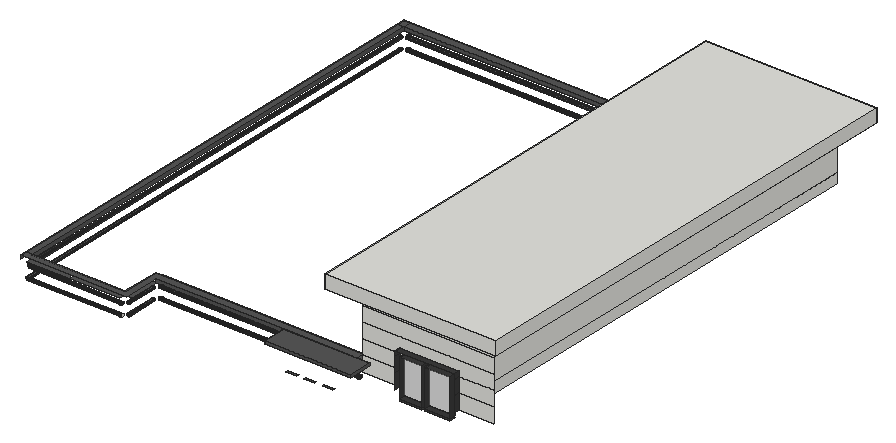
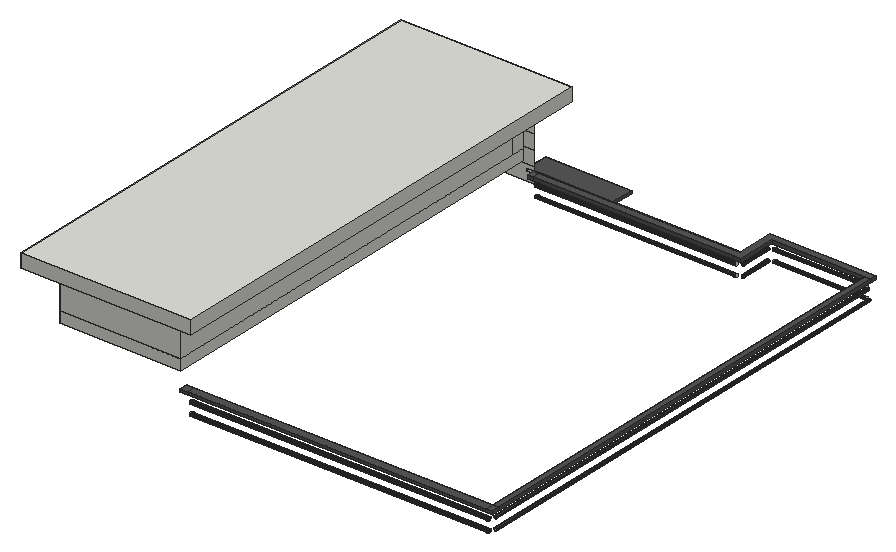
# SketchUp Ruby script. Lengths in inches.
U = 1.inch
M = Sketchup.active_model
def pt(a) = Geom::Point3d.new(a.map { |v| v * U })
def face(e, loops, mat)
  f = e.add_face(loops[0].map { |a| pt(a) })
  loops[1..].each { |l| e.add_face(l.map { |a| pt(a) }).erase! }
  f.material = f.back_material = mat if mat
  f
end
# faces: each face lists its corners as indices into pts; further lists are holes
def faces(e, pts, list, mat = nil) = list.each { |f| face(e, (f[0].is_a?(Array) ? f : [f]).map { |l| l.map { |i| pts[i] } }, mat) }
# xy, xz, yz: faces in a plane at the given z, y or x. An outline is a flat list of corners, or four numbers for a rectangle; further outlines are holes
def ring(l) = l.size == 4 ? [[l[0], l[1]], [l[2], l[1]], [l[2], l[3]], [l[0], l[3]]] : l.each_slice(2).to_a
def flat(e, list, mat, &to3) = list.each { |f| face(e, (f[0].is_a?(Array) ? f : [f]).map { |l| ring(l).map { |u, v| to3.(u, v) } }, mat) }
def xy(e, z, list, mat = nil) = flat(e, list, mat) { |x, y| [x, y, z] }
def xz(e, y, list, mat = nil) = flat(e, list, mat) { |x, z| [x, y, z] }
def yz(e, x, list, mat = nil) = flat(e, list, mat) { |y, z| [x, y, z] }
def lines(e, pts, list) = list.each { |a, b| e.add_line(pt(pts[a]), pt(pts[b])) }
# prism: a flat outline (further loops are holes) pulled along v
def prism(e, loops, v, mat = nil)
  f = face(e, loops, mat); d = Geom::Vector3d.new(v.map { |x| x * U })
  f.pushpull(f.normal.samedirection?(d) ? d.length : -d.length)
end
def box(e, o, s, mat = nil) = prism(e, [[o, [o[0] + s[0], o[1], o[2]], [o[0] + s[0], o[1] + s[1], o[2]], [o[0], o[1] + s[1], o[2]]]], [0, 0, s[2]], mat)
def at(x, y, z, deg = 0) = Geom::Transformation.translation(pt([x, y, z])) * Geom::Transformation.rotation(ORIGIN, Z_AXIS, deg.degrees)
def axes(o, x, y, z) = Geom::Transformation.new([*x, 0, *y, 0, *z, 0, *pt(o).to_a, 1])
def part(name) = M.definitions.add(name)
# library, detail: a bought-in or finely detailed component or shape, given as its bounding box
def library(name, o, s) = part(name).tap { |d| box(d.entities, o, s) }
def detail(e, o, s) = box(e.add_group.entities, o, s)
def put(e, d, t, mat = nil) = e.add_instance(d, t).tap { |i| i.material = mat if mat }
def group(e, t, mat = nil) = e.add_group.tap { |g| g.transformation = t; g.material = mat if mat }.entities
root = M.entities
M.materials.add("[Color M06]").color = [86, 86, 86]
M.materials.add("[Color M07]").color = [58, 58, 58]
M.materials.add("[Translucent Glass Gray]").color = [128, 128, 128]
M.materials["[Translucent Glass Gray]"].alpha = 0.5
M.materials.add("[Wood Fence]").color = [142, 67, 30]
xy(root,343.87,[[283.87,125.84,295.81,128.03],[304,125.84,315.93,128.03],[324.62,125.84,336.56,128.03]],"[Color M06]")
xy(root,347.76,[[3.85,111.5,4.24,637.4375]],"[Color M06]")
xy(root,348.22,[[399.25,141.23,424.3125,147.79],[427.08,141.23,456,147.79]],"[Color M07]")
xy(root,350.29,[[399.25,141.23,424.3125,147.79],[427.08,141.23,456,147.79]],"[Color M07]")
xy(root,366,[[206.23,639.05,209.79,643.61]])
xy(root,366.125,[[[0,113.71,7.24,637.4375],[1.32,218.77,6.25,221.71],[1.32,568.77,6.25,571.71],[1.32,483.08,6.25,486.02],[1.32,393.08,6.25,396.02],[1.32,307.08,6.25,310.02]],[346.24,147.79,352,156.79],[112.36,149.1,120,156.79],[0,637.4375,7.24,646.4375],[[7.24,637.4375,343.33,646.4375],[285.6,637.86,289.17,643.61],[92.17,637.86,95.73,643.55]],
  [343.33,637.4375,352,646.4375]])
xy(root,366.125,[[[7.24,106.4375,112.36,113.71],[52.52,108.5,56.02,112.75]],[112.36,113.71,120,149.1],[120,147.79,346.24,156.79]],"[Color M06]")
xy(root,367.0625,[[266.86,121.03,269.98,140.23],[269.98,128.03,352,140.23]])
xy(root,367.0625,[[263.17,121.03,263.17,147.79,360.875,147.79,360.875,128.03,352,128.03,352,140.23,266.86,140.23,266.86,121.03],[269.98,121.03,360.875,128.03]],"[Color M06]")
xy(root,370,[[0,106.4375,120,106.4375,120,147.79,346.24,147.79,346.24,156.79,112.36,156.79,112.36,113.71,0,113.71],[0,113.71,7.24,637.4375],[263.17,121.03,360.875,147.79],[346.24,147.79,352,156.79],[0,637.4375,7.24,646.4375],
  [7.24,637.4375,343.33,646.4375],[343.33,637.4375,352,646.4375]],"[Color M06]")
xy(root,392.08,[[399.25,141.23,424.3125,147.79],[427.08,141.23,428.9,147.79],[428.9,141.23,456,147.79]],"[Color M07]")
xy(root,394,[[358,155.92,494,637.4375]])
xy(root,397.01,[[394.33,141.23,460.92,147.79]],"[Color M07]")
xy(root,435.0625,[[358,155.92,494,637.4375]])
xy(root,441.0625,[[352,147.79,500,646.4375]])
xy(root,441.0625,[[[325.625,127.92,517.6875,664.0625],[352,147.79,500,646.4375]]],"[Wood Fence]")
xy(root,455.875,[[325.625,127.92,517.6875,664.0625]])
xz(root,111.5,[[4.17,344.78,4.55,344.875,4.9,345.0625,5.18,345.33,5.38,345.67,5.49,346.04,5.5,346.44,5.41,346.82,5.22,347.16,4.95,347.44,4.61,347.65,4.24,347.76,3.85,347.76,3.47,347.67,3.125,347.48,2.84,347.21,2.64,346.88,2.53,346.5,2.52,346.11,2.61,345.73,2.8,345.39,3.07,345.1,3.4,344.9,3.78,344.79]])
xz(root,113.71,[[116.05,345.98,116.46,346,116.84,346.125,117.1875,346.35,117.46,346.65,117.65,347.01,117.73,347.41,117.71,347.82,117.58,348.21,117.36,348.55,117.06,348.82,116.69,349.01,116.3,349.09,115.89,349.07,115.5,348.95,115.16,348.72,114.89,348.42,114.7,348.06,114.62,347.66,114.64,347.25,114.76,346.86,114.98,346.52,115.29,346.25,115.65,346.0625],[116.05,358.29,116.46,358.3125,116.84,358.4375,117.1875,358.66,117.46,358.96,117.65,359.33,117.73,359.73,117.71,360.13,117.58,360.52,117.36,360.86,117.06,361.14,116.69,361.32,116.3,361.41,115.89,361.39,115.5,361.26,115.16,361.04,114.89,360.73,114.7,360.37,114.62,359.97,114.64,359.56,114.76,359.18,114.98,358.83,115.29,358.5625,115.65,358.375]])
xz(root,113.71,[[7.24,366.125,112.36,370]],"[Color M06]")
xz(root,121.03,[[263.17,367.0625,360.875,370]],"[Color M06]")
xz(root,127.92,[[325.625,441.0625,517.6875,455.875]])
xz(root,147.79,[[352,357.85,394.33,357.85,394.33,374.6,352,374.6,352,370,360.875,370,360.875,367.0625,352,367.0625],[460.92,357.85,500,374.6],[346.24,366.125,352,367.0625],[263.17,367.0625,346.24,370],[346.24,367.0625,352,370],
  [352,367.0625,360.875,370],[352,374.6,394.33,391.35],[460.92,374.6,500,391.35],[352,391.35,394.33,391.35,394.33,397.01,460.92,397.01,460.92,391.35,500,391.35,500,408.1,352,408.1],[352,408.1,500,424.0625],
  [352,424.0625,500,441.0625]])
xz(root,147.79,[[120,366.125,346.24,366.125,346.24,367.0625,263.17,367.0625,263.17,370,120,370]],"[Color M06]")
xz(root,147.79,[[399.25,350.29,424.3125,392.08],[427.08,350.29,456,392.08]],"[Translucent Glass Gray]")
xz(root,148.83,[[116.05,358.29,115.65,358.375,115.29,358.5625,114.98,358.83,114.76,359.18,114.64,359.56,114.62,359.97,114.7,360.37,114.89,360.73,115.16,361.04,115.5,361.26,115.89,361.39,116.3,361.41,116.69,361.32,117.06,361.14,117.36,360.86,117.58,360.52,117.71,360.13,117.73,359.73,117.65,359.33,117.46,358.96,117.1875,358.66,116.84,358.4375,116.46,358.3125]])
xz(root,155.92,[[358,382,494,394],[358,394,494,424.0625],[358,424.0625,494,435.0625]])
xz(root,156.79,[[112.36,366.125,120,370],[120,366.125,346.24,370],[346.24,366.125,352,370]],"[Color M06]")
xz(root,637.4375,[[4.17,344.78,3.78,344.79,3.4,344.9,3.07,345.1,2.8,345.39,2.61,345.73,2.52,346.11,2.53,346.5,2.64,346.88,2.84,347.21,3.125,347.48,3.47,347.67,3.85,347.76,4.24,347.76,4.61,347.65,4.95,347.44,5.22,347.16,5.41,346.82,5.5,346.44,5.49,346.04,5.38,345.67,5.18,345.33,4.9,345.0625,4.55,344.875],[4.17,357.09,3.78,357.1,3.4,357.21,3.07,357.42,2.8,357.7,2.61,358.04,2.52,358.42,2.53,358.82,2.64,359.19,2.84,359.53,3.125,359.8,3.47,359.98,3.85,360.08,4.24,360.07,4.61,359.96,4.95,359.75,5.22,359.47,5.41,359.13,5.5,358.75,5.49,358.36,5.38,357.98,5.18,357.65,4.9,357.375,4.55,357.1875],[358,382,494,394],[358,394,494,424.0625],[358,424.0625,494,435.0625]])
xz(root,637.4375,[[7.24,366.125,343.33,370],[343.33,366.125,352,370]],"[Color M06]")
xz(root,646.4375,[[0,366.125,7.24,370],[7.24,366.125,343.33,370],[343.33,366.125,352,370]],"[Color M06]")
xz(root,664.0625,[[325.625,441.0625,517.6875,455.875]])
yz(root,0,[[106.4375,366.125,113.71,370],[113.71,366.125,637.4375,370],[637.4375,366.125,646.4375,370]],"[Color M06]")
yz(root,7.24,[[110.32,345.27,109.9375,345.32,109.57,345.47,109.26,345.71,109.03,346.02,108.875,346.38,108.82,346.77,108.875,347.16,109.03,347.52,109.26,347.83,109.57,348.07,109.9375,348.22,110.32,348.27,110.71,348.22,111.07,348.07,111.38,347.83,111.625,347.52,111.77,347.16,111.82,346.77,111.77,346.38,111.625,346.02,111.38,345.71,111.07,345.47,110.71,345.32],[110.32,357.9,109.9375,357.95,109.57,358.1,109.26,358.34,109.03,358.65,108.875,359.01,108.82,359.4,108.875,359.78,109.03,360.15,109.26,360.46,109.57,360.69,109.9375,360.84,110.32,360.9,110.71,360.84,111.07,360.69,111.38,360.46,111.625,360.15,111.77,359.78,111.82,359.4,111.77,359.01,111.625,358.65,111.38,358.34,111.07,358.1,110.71,357.95]])
yz(root,7.24,[[113.71,366.125,637.4375,370]],"[Color M06]")
yz(root,112.11,[[110.32,345.27,110.71,345.32,111.07,345.47,111.38,345.71,111.625,346.02,111.77,346.38,111.82,346.77,111.77,347.16,111.625,347.52,111.38,347.83,111.07,348.07,110.71,348.22,110.32,348.27,109.9375,348.22,109.57,348.07,109.26,347.83,109.03,347.52,108.875,347.16,108.82,346.77,108.875,346.38,109.03,346.02,109.26,345.71,109.57,345.47,109.9375,345.32]])
yz(root,112.36,[[113.71,366.125,156.79,370]],"[Color M06]")
yz(root,120,[[152.72,347.12,152.32,347.17,151.94,347.33,151.62,347.58,151.37,347.9,151.21,348.28,151.16,348.68,151.21,349.09,151.37,349.46,151.62,349.79,151.94,350.04,152.32,350.19,152.72,350.25,153.125,350.19,153.5,350.04,153.83,349.79,154.07,349.46,154.23,349.09,154.28,348.68,154.23,348.28,154.07,347.9,153.83,347.58,153.5,347.33,153.125,347.17],[152.72,358.93,152.32,358.99,151.94,359.14,151.62,359.39,151.37,359.71,151.21,360.09,151.16,360.5,151.21,360.9,151.37,361.28,151.62,361.6,151.94,361.85,152.32,362,152.72,362.06,153.125,362,153.5,361.85,153.83,361.6,154.07,361.28,154.23,360.9,154.28,360.5,154.23,360.09,154.07,359.71,153.83,359.39,153.5,359.14,153.125,358.99]])
yz(root,263.17,[[121.03,367.0625,147.79,370]],"[Color M06]")
yz(root,325.625,[[127.92,441.0625,664.0625,455.875]])
yz(root,343.33,[[641.59,343.41,642.0625,343.48,642.5,343.66,642.875,343.94,643.16,344.32,643.35,344.76,643.41,345.23,643.35,345.7,643.16,346.13,642.875,346.51,642.5,346.8,642.0625,346.98,641.59,347.04,641.125,346.98,640.6875,346.8,640.3125,346.51,640.03,346.13,639.84,345.7,639.78,345.23,639.84,344.76,640.03,344.32,640.3125,343.94,640.6875,343.66,641.125,343.48]])
yz(root,352,[[637.4375,366.125,646.4375,370]])
yz(root,358,[[155.92,382,637.4375,394],[155.92,394,170.17,424.0625],[170.17,394,637.4375,424.0625],[155.92,424.0625,170.17,435.0625],[170.17,424.0625,637.4375,435.0625]])
yz(root,360.875,[[121.03,367.0625,147.79,370]],"[Color M06]")
yz(root,394.33,[[141.23,357.85,147.79,374.6],[141.23,374.6,147.79,391.35],[141.23,391.35,147.79,397.01]],"[Color M07]")
yz(root,399.25,[[141.23,350.29,147.79,392.08]],"[Color M07]")
yz(root,424.3125,[[141.23,350.29,147.79,392.08]],"[Color M07]")
yz(root,427.08,[[141.23,350.29,147.79,392.08]],"[Color M07]")
yz(root,456,[[141.23,350.29,147.79,392.08]],"[Color M07]")
yz(root,460.92,[[141.23,357.85,147.79,374.6],[141.23,374.6,147.79,391.35],[141.23,391.35,147.79,397.01]],"[Color M07]")
yz(root,494,[[155.92,382,637.4375,394],[155.92,394,637.4375,424.0625],[155.92,424.0625,637.4375,435.0625]])
yz(root,517.6875,[[127.92,441.0625,664.0625,455.875]])
p = [[343.33,641.59,343.41],[343.33,641.125,343.48],[7.24,641.125,343.48],[7.24,641.59,343.41],[343.33,642.0625,343.48],[7.24,642.0625,343.48],
  [343.33,640.6875,343.66],[7.24,640.6875,343.66],[343.33,642.5,343.66],[7.24,642.5,343.66],[343.33,640.3125,343.94],[7.24,640.3125,343.94],
  [343.33,642.875,343.94],[7.24,642.875,343.94],[343.33,640.03,344.32],[7.24,640.03,344.32],[343.33,643.16,344.32],[7.24,643.16,344.32],
  [343.33,639.84,344.76],[7.24,639.84,344.76],[343.33,643.35,344.76],[7.24,643.35,344.76],[3.4,637.4375,344.9],[3.78,637.4375,344.79],
  [3.78,111.5,344.79],[3.4,111.5,344.9],[4.17,637.4375,344.78],[4.17,111.5,344.78],[4.55,637.4375,344.875],[4.55,111.5,344.875],
  [343.33,639.78,345.23],[7.24,639.78,345.23],[343.33,643.41,345.23],[7.24,643.41,345.23],[3.07,637.4375,345.1],[3.07,111.5,345.1],
  [4.9,637.4375,345.0625],[4.9,111.5,345.0625],[2.8,637.4375,345.39],[2.8,111.5,345.39],[5.18,637.4375,345.33],[5.18,111.5,345.33],
  [343.33,639.84,345.7],[7.24,639.84,345.7],[343.33,643.35,345.7],[7.24,643.35,345.7],[7.24,109.57,345.47],[7.24,109.9375,345.32],
  [112.11,109.9375,345.32],[112.11,109.57,345.47],[7.24,110.32,345.27],[112.11,110.32,345.27],[7.24,110.71,345.32],[112.11,110.71,345.32],
  [7.24,111.07,345.47],[112.11,111.07,345.47],[5.38,637.4375,345.67],[5.38,111.5,345.67],[2.61,637.4375,345.73],[2.61,111.5,345.73],
  [7.24,109.26,345.71],[112.11,109.26,345.71],[7.24,111.38,345.71],[112.11,111.38,345.71],[7.24,109.03,346.02],[112.11,109.03,346.02],
  [7.24,111.625,346.02],[112.11,111.625,346.02],[2.52,637.4375,346.11],[2.52,111.5,346.11],[5.49,637.4375,346.04],[5.49,111.5,346.04],
  [343.33,640.03,346.13],[7.24,640.03,346.13],[343.33,643.16,346.13],[7.24,643.16,346.13],[7.24,108.875,346.38],[112.11,108.875,346.38],
  [5.5,637.4375,346.44],[5.5,111.5,346.44],[7.24,111.77,346.38],[112.11,111.77,346.38],[116.05,113.71,345.98],[115.65,113.71,346.0625],
  [115.65,149.1,346.0625],[116.05,149.1,345.98],[116.46,113.71,346],[116.46,149.1,346],[116.84,113.71,346.125],[116.84,149.1,346.125],
  [2.53,637.4375,346.5],[2.53,111.5,346.5],[115.29,113.71,346.25],[115.29,149.1,346.25],[117.1875,113.71,346.35],[117.1875,149.1,346.35],
  [343.33,640.3125,346.51],[7.24,640.3125,346.51],[343.33,642.875,346.51],[7.24,642.875,346.51],[114.98,113.71,346.52],[114.98,149.1,346.52],
  [117.46,113.71,346.65],[117.46,149.1,346.65],[7.24,108.82,346.77],[112.11,108.82,346.77],[5.41,637.4375,346.82],[5.41,111.5,346.82],
  [7.24,111.82,346.77],[112.11,111.82,346.77],[2.64,637.4375,346.88],[2.64,111.5,346.88],[114.76,113.71,346.86],[114.76,149.1,346.86],
  [343.33,640.6875,346.8],[7.24,640.6875,346.8],[343.33,642.5,346.8],[7.24,642.5,346.8],[117.65,113.71,347.01],[117.65,149.1,347.01],
  [7.24,108.875,347.16],[112.11,108.875,347.16],[5.22,637.4375,347.16],[5.22,111.5,347.16],[7.24,111.77,347.16],[112.11,111.77,347.16],
  [343.33,641.125,346.98],[7.24,641.125,346.98],[343.33,642.0625,346.98],[7.24,642.0625,346.98],[2.84,637.4375,347.21],[2.84,111.5,347.21],
  [114.64,113.71,347.25],[114.64,149.1,347.25],[117.73,113.71,347.41],[117.73,149.1,347.41],[343.33,641.59,347.04],[7.24,641.59,347.04],
  [120,152.32,347.17],[120,152.72,347.12],[346.24,152.72,347.12],[346.24,152.32,347.17],[120,153.125,347.17],[346.24,153.125,347.17],
  [7.24,109.03,347.52],[112.11,109.03,347.52],[3.125,637.4375,347.48],[3.125,111.5,347.48],[4.95,637.4375,347.44],[4.95,111.5,347.44],
  [7.24,111.625,347.52],[112.11,111.625,347.52],[120,151.94,347.33],[346.24,151.94,347.33],[120,153.5,347.33],[346.24,153.5,347.33],
  [114.62,113.71,347.66],[114.62,149.1,347.66],[120,151.62,347.58],[346.24,151.62,347.58],[120,153.83,347.58],[346.24,153.83,347.58],
  [4.61,637.4375,347.65],[4.61,111.5,347.65],[117.71,113.71,347.82],[117.71,149.1,347.82],[7.24,109.26,347.83],[112.11,109.26,347.83],
  [7.24,111.38,347.83],[112.11,111.38,347.83],[3.47,637.4375,347.67],[3.47,111.5,347.67],[4.24,637.4375,347.76],[4.24,111.5,347.76],
  [120,151.37,347.9],[346.24,151.37,347.9],[120,154.07,347.9],[346.24,154.07,347.9],[3.85,637.4375,347.76],[3.85,111.5,347.76],
  [114.7,113.71,348.06],[114.7,149.1,348.06],[7.24,109.57,348.07],[112.11,109.57,348.07],[7.24,111.07,348.07],[112.11,111.07,348.07],
  [117.58,113.71,348.21],[117.58,149.1,348.21],[120,151.21,348.28],[346.24,151.21,348.28],[120,154.23,348.28],[346.24,154.23,348.28],
  [7.24,109.9375,348.22],[112.11,109.9375,348.22],[7.24,110.71,348.22],[112.11,110.71,348.22],[114.89,113.71,348.42],[114.89,149.1,348.42],
  [7.24,110.32,348.27],[112.11,110.32,348.27],[117.36,113.71,348.55],[117.36,149.1,348.55],[120,151.16,348.68],[346.24,151.16,348.68],
  [120,154.28,348.68],[346.24,154.28,348.68],[115.16,113.71,348.72],[115.16,149.1,348.72],[117.06,113.71,348.82],[117.06,149.1,348.82],
  [115.5,113.71,348.95],[115.5,149.1,348.95],[120,151.21,349.09],[346.24,151.21,349.09],[120,154.23,349.09],[346.24,154.23,349.09],
  [116.69,113.71,349.01],[116.69,149.1,349.01],[115.89,113.71,349.07],[115.89,149.1,349.07],[116.3,113.71,349.09],[116.3,149.1,349.09],
  [120,151.37,349.46],[346.24,151.37,349.46],[120,154.07,349.46],[346.24,154.07,349.46],[120,151.62,349.79],[346.24,151.62,349.79],
  [120,153.83,349.79],[346.24,153.83,349.79],[120,151.94,350.04],[346.24,151.94,350.04],[120,153.5,350.04],[346.24,153.5,350.04],
  [120,152.32,350.19],[346.24,152.32,350.19],[120,153.125,350.19],[346.24,153.125,350.19],[120,152.72,350.25],[346.24,152.72,350.25],
  [343.33,641.125,355.91],[343.33,640.6875,356.09],[7.24,640.6875,356.09],[7.24,641.125,355.91],[343.33,641.59,355.85],[7.24,641.59,355.85],
  [343.33,642.0625,355.91],[7.24,642.0625,355.91],[343.33,642.5,356.09],[7.24,642.5,356.09],[343.33,640.3125,356.38],[7.24,640.3125,356.38],
  [343.33,642.875,356.38],[7.24,642.875,356.38],[343.33,640.03,356.76],[7.24,640.03,356.76],[343.33,643.16,356.76],[7.24,643.16,356.76],
  [343.33,639.84,357.19],[7.24,639.84,357.19],[343.33,643.35,357.19],[7.24,643.35,357.19],[3.4,637.4375,357.21],[3.78,637.4375,357.1],
  [3.78,113.71,357.1],[3.4,113.71,357.21],[4.17,637.4375,357.09],[4.17,113.71,357.09],[4.55,637.4375,357.1875],[4.55,113.71,357.1875],
  [3.07,637.4375,357.42],[3.07,113.71,357.42],[4.9,637.4375,357.375],[4.9,113.71,357.375],[343.33,639.78,357.66],[7.24,639.78,357.66],
  [343.33,643.41,357.66],[7.24,643.41,357.66],[2.8,637.4375,357.7],[2.8,113.71,357.7],[5.18,637.4375,357.65],[5.18,113.71,357.65],
  [5.38,637.4375,357.98],[5.38,113.71,357.98],[2.61,637.4375,358.04],[2.61,113.71,358.04],[343.33,639.84,358.13],[7.24,639.84,358.13],
  [343.33,643.35,358.13],[7.24,643.35,358.13],[7.24,109.57,358.1],[7.24,109.9375,357.95],[112.36,109.9375,357.95],[112.36,109.57,358.1],
  [7.24,110.32,357.9],[112.36,110.32,357.9],[7.24,110.71,357.95],[112.36,110.71,357.95],[7.24,111.07,358.1],[112.36,111.07,358.1],
  [2.52,637.4375,358.42],[2.52,113.71,358.42],[5.49,637.4375,358.36],[5.49,113.71,358.36],[7.24,109.26,358.34],[112.36,109.26,358.34],
  [7.24,111.38,358.34],[112.36,111.38,358.34],[343.33,640.03,358.57],[7.24,640.03,358.57],[343.33,643.16,358.57],[7.24,643.16,358.57],
  [7.24,109.03,358.65],[112.36,109.03,358.65],[7.24,111.625,358.65],[112.36,111.625,358.65],[116.05,113.71,358.29],[115.65,113.71,358.375],
  [115.65,148.83,358.375],[116.05,148.83,358.29],[116.46,113.71,358.3125],[116.46,148.83,358.3125],[116.84,113.71,358.4375],[116.84,148.83,358.4375],
  [2.53,637.4375,358.82],[2.53,113.71,358.82],[5.5,637.4375,358.75],[5.5,113.71,358.75],[115.29,113.71,358.5625],[115.29,148.83,358.5625],
  [117.1875,113.71,358.66],[117.1875,148.83,358.66],[7.24,108.875,359.01],[112.36,108.875,359.01],[7.24,111.77,359.01],[112.36,111.77,359.01],
  [114.98,113.71,358.83],[114.98,148.83,358.83],[343.33,640.3125,358.95],[7.24,640.3125,358.95],[343.33,642.875,358.95],[7.24,642.875,358.95],
  [5.41,637.4375,359.13],[5.41,113.71,359.13],[117.46,113.71,358.96],[117.46,148.83,358.96],[2.64,637.4375,359.19],[2.64,113.71,359.19],
  [114.76,113.71,359.18],[114.76,148.83,359.18],[120,152.32,358.99],[120,152.72,358.93],[346.24,152.72,358.93],[346.24,152.32,358.99],
  [120,153.125,358.99],[346.24,153.125,358.99],[343.33,640.6875,359.23],[7.24,640.6875,359.23],[343.33,642.5,359.23],[7.24,642.5,359.23],
  [7.24,108.82,359.4],[112.36,108.82,359.4],[7.24,111.82,359.4],[112.36,111.82,359.4],[117.65,113.71,359.33],[117.65,148.83,359.33],
  [120,151.94,359.14],[346.24,151.94,359.14],[120,153.5,359.14],[346.24,153.5,359.14],[5.22,637.4375,359.47],[5.22,113.71,359.47],
  [120,151.62,359.39],[346.24,151.62,359.39],[120,153.83,359.39],[346.24,153.83,359.39],[2.84,637.4375,359.53],[2.84,113.71,359.53],
  [114.64,113.71,359.56],[114.64,148.83,359.56],[343.33,641.125,359.41],[7.24,641.125,359.41],[343.33,642.0625,359.41],[7.24,642.0625,359.41],
  [117.73,113.71,359.73],[117.73,148.83,359.73],[7.24,108.875,359.78],[112.36,108.875,359.78],[7.24,111.77,359.78],[112.36,111.77,359.78],
  [120,151.37,359.71],[346.24,151.37,359.71],[120,154.07,359.71],[346.24,154.07,359.71],[343.33,641.59,359.48],[7.24,641.59,359.48],
  [3.125,637.4375,359.8],[3.125,113.71,359.8],[4.95,637.4375,359.75],[4.95,113.71,359.75],[114.62,113.71,359.97],[114.62,148.83,359.97],
  [117.71,113.71,360.13],[117.71,148.83,360.13],[120,151.21,360.09],[346.24,151.21,360.09],[120,154.23,360.09],[346.24,154.23,360.09],
  [7.24,109.03,360.15],[112.36,109.03,360.15],[7.24,111.625,360.15],[112.36,111.625,360.15],[3.47,637.4375,359.98],[3.47,113.71,359.98],
  [4.61,637.4375,359.96],[4.61,113.71,359.96],[3.85,637.4375,360.08],[3.85,113.71,360.08],[4.24,637.4375,360.07],[4.24,113.71,360.07],
  [114.7,113.71,360.37],[114.7,148.83,360.37],[7.24,109.26,360.46],[112.36,109.26,360.46],[7.24,111.38,360.46],[112.36,111.38,360.46],
  [117.58,113.71,360.52],[117.58,148.83,360.52],[120,151.16,360.5],[346.24,151.16,360.5],[120,154.28,360.5],[346.24,154.28,360.5],
  [114.89,113.71,360.73],[114.89,148.83,360.73],[7.24,109.57,360.69],[112.36,109.57,360.69],[7.24,111.07,360.69],[112.36,111.07,360.69],
  [117.36,113.71,360.86],[117.36,148.83,360.86],[120,151.21,360.9],[346.24,151.21,360.9],[120,154.23,360.9],[346.24,154.23,360.9],
  [7.24,109.9375,360.84],[112.36,109.9375,360.84],[7.24,110.71,360.84],[112.36,110.71,360.84],[115.16,113.71,361.04],[115.16,148.83,361.04],
  [7.24,110.32,360.9],[112.36,110.32,360.9],[117.06,113.71,361.14],[117.06,148.83,361.14],[120,151.37,361.28],[346.24,151.37,361.28],
  [120,154.07,361.28],[346.24,154.07,361.28],[115.5,113.71,361.26],[115.5,148.83,361.26],[116.69,113.71,361.32],[116.69,148.83,361.32],
  [115.89,113.71,361.39],[115.89,148.83,361.39],[116.3,113.71,361.41],[116.3,148.83,361.41],[120,151.62,361.6],[346.24,151.62,361.6],
  [120,153.83,361.6],[346.24,153.83,361.6],[120,151.94,361.85],[346.24,151.94,361.85],[120,153.5,361.85],[346.24,153.5,361.85],
  [120,152.32,362],[346.24,152.32,362],[120,153.125,362],[346.24,153.125,362],[120,152.72,362.06],[346.24,152.72,362.06],
  [494,637.4375,435.0625],[494,637.4375,441.0625],[358,637.4375,435.0625],[358,637.4375,441.0625],[494,155.92,435.0625],[494,155.92,441.0625],
  [358,170.17,435.0625],[358,170.17,441.0625]]
faces(root,p,[[0,1,2,3],[4,0,3,5],[1,6,7,2],[8,4,5,9],[6,10,11,7],[12,8,9,13],[10,14,15,11],[16,12,13,17],
  [14,18,19,15],[20,16,17,21],[22,23,24,25],[23,26,27,24],[26,28,29,27],[18,30,31,19],[32,20,21,33],[34,22,25,35],
  [28,36,37,29],[38,34,35,39],[36,40,41,37],[30,42,43,31],[44,32,33,45],[46,47,48,49],[47,50,51,48],[50,52,53,51],
  [52,54,55,53],[40,56,57,41],[58,38,39,59],[60,46,49,61],[54,62,63,55],[64,60,61,65],[62,66,67,63],[68,58,59,69],
  [56,70,71,57],[42,72,73,43],[74,44,45,75],[76,64,65,77],[70,78,79,71],[66,80,81,67],[82,83,84,85],[86,82,85,87],
  [88,86,87,89],[90,68,69,91],[83,92,93,84],[94,88,89,95],[72,96,97,73],[98,74,75,99],[92,100,101,93],[102,94,95,103],
  [104,76,77,105],[78,106,107,79],[80,108,109,81],[110,90,91,111],[100,112,113,101],[96,114,115,97],[116,98,99,117],[118,102,103,119],
  [120,104,105,121],[106,122,123,107],[108,124,125,109],[114,126,127,115],[128,116,117,129],[130,110,111,131],[112,132,133,113],[134,118,119,135],
  [126,136,137,127],[136,128,129,137],[138,139,140,141],[139,142,143,140],[144,120,121,145],[146,130,131,147],[122,148,149,123],[124,150,151,125],
  [152,138,141,153],[142,154,155,143],[132,156,157,133],[158,152,153,159],[154,160,161,155],[148,162,163,149],[164,134,135,165],[166,144,145,167],
  [150,168,169,151],[170,146,147,171],[162,172,173,163],[174,158,159,175],[160,176,177,161],[178,170,171,179],[156,180,181,157],[182,166,167,183],
  [168,184,185,169],[186,164,165,187],[188,174,175,189],[176,190,191,177],[192,182,183,193],[184,194,195,185],[180,196,197,181],[198,192,193,199],
  [194,198,199,195],[200,186,187,201],[202,188,189,203],[190,204,205,191],[196,206,207,197],[208,200,201,209],[206,210,211,207],[212,202,203,213],
  [204,214,215,205],[216,208,209,217],[210,218,219,211],[220,216,217,221],[218,220,221,219],[222,212,213,223],[214,224,225,215],[226,222,223,227],
  [224,228,229,225],[230,226,227,231],[228,232,233,229],[234,230,231,235],[232,236,237,233],[238,234,235,239],[236,238,239,237],[240,241,242,243],
  [244,240,243,245],[246,244,245,247],[248,246,247,249],[241,250,251,242],[252,248,249,253],[250,254,255,251],[256,252,253,257],[254,258,259,255],
  [260,256,257,261],[262,263,264,265],[263,266,267,264],[266,268,269,267],[270,262,265,271],[268,272,273,269],[258,274,275,259],[276,260,261,277],
  [278,270,271,279],[272,280,281,273],[280,282,283,281],[284,278,279,285],[274,286,287,275],[288,276,277,289],[290,291,292,293],[291,294,295,292],
  [294,296,297,295],[296,298,299,297],[300,284,285,301],[282,302,303,283],[304,290,293,305],[298,306,307,299],[286,308,309,287],[310,288,289,311],
  [312,304,305,313],[306,314,315,307],[316,317,318,319],[320,316,319,321],[322,320,321,323],[324,300,301,325],[302,326,327,303],[317,328,329,318],
  [330,322,323,331],[332,312,313,333],[314,334,335,315],[328,336,337,329],[308,338,339,309],[340,310,311,341],[326,342,343,327],[344,330,331,345],
  [346,324,325,347],[336,348,349,337],[350,351,352,353],[351,354,355,352],[338,356,357,339],[358,340,341,359],[360,332,333,361],[334,362,363,335],
  [364,344,345,365],[366,350,353,367],[354,368,369,355],[342,370,371,343],[372,366,367,373],[368,374,375,369],[376,346,347,377],[348,378,379,349],
  [356,380,381,357],[382,358,359,383],[384,364,365,385],[386,360,361,387],[362,388,389,363],[390,372,373,391],[374,392,393,375],[380,394,395,381],
  [394,382,383,395],[396,376,377,397],[370,398,399,371],[378,400,401,379],[402,384,385,403],[404,390,391,405],[392,406,407,393],[408,386,387,409],
  [388,410,411,389],[412,396,397,413],[398,414,415,399],[416,412,413,417],[414,418,419,415],[400,420,421,401],[422,408,409,423],[410,424,425,411],
  [418,416,417,419],[426,402,403,427],[428,404,405,429],[406,430,431,407],[420,432,433,421],[434,422,423,435],[424,436,437,425],[438,426,427,439],
  [440,428,429,441],[430,442,443,431],[444,434,435,445],[436,446,447,437],[432,448,449,433],[450,444,445,451],[446,450,451,447],[452,438,439,453],
  [454,440,441,455],[442,456,457,443],[448,458,459,449],[460,452,453,461],[458,462,463,459],[464,460,461,465],[466,454,455,467],[456,468,469,457],
  [462,464,465,463],[470,466,467,471],[468,472,473,469],[474,470,471,475],[472,476,477,473],[478,474,475,479],[476,478,479,477]],"[Color M06]")
lines(root,p,[[480,481],[482,483],[484,485],[486,487]])
